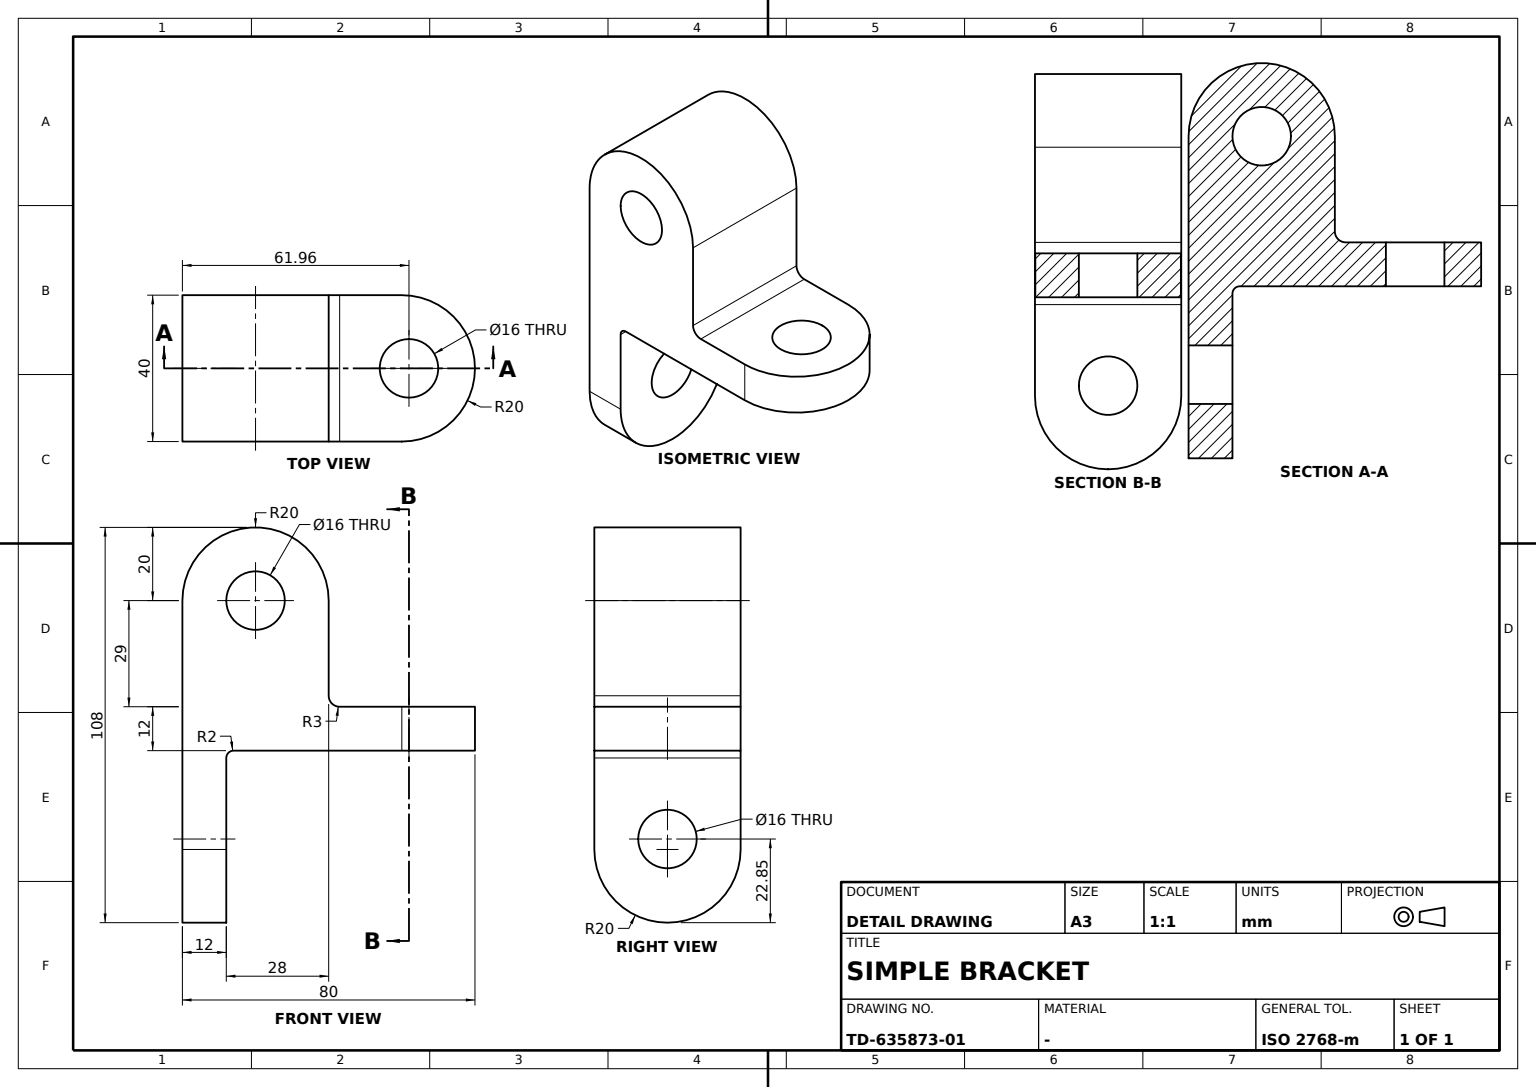
ISO-10303-21;
HEADER;
FILE_DESCRIPTION((''),'2;1');
FILE_NAME('','',(''),(''),'','','');
FILE_SCHEMA(('AUTOMOTIVE_DESIGN'));
ENDSEC;
DATA;
#1=APPLICATION_CONTEXT('');
#2=PRODUCT_CONTEXT('',#1,'mechanical');
#3=PRODUCT('','','',(#2));
#4=PRODUCT_DEFINITION_FORMATION('','',#3);
#5=PRODUCT_DEFINITION_CONTEXT('',#1,'design');
#6=PRODUCT_DEFINITION('','',#4,#5);
#7=PRODUCT_DEFINITION_SHAPE('','',#6);
#8=(LENGTH_UNIT()NAMED_UNIT(*)SI_UNIT(.MILLI.,.METRE.));
#9=(NAMED_UNIT(*)PLANE_ANGLE_UNIT()SI_UNIT($,.RADIAN.));
#10=(NAMED_UNIT(*)SI_UNIT($,.STERADIAN.)SOLID_ANGLE_UNIT());
#11=UNCERTAINTY_MEASURE_WITH_UNIT(LENGTH_MEASURE(1.E-05),#8,'distance_accuracy_value','');
#12=(GEOMETRIC_REPRESENTATION_CONTEXT(3)GLOBAL_UNCERTAINTY_ASSIGNED_CONTEXT((#11))GLOBAL_UNIT_ASSIGNED_CONTEXT((#8,#9,#10))REPRESENTATION_CONTEXT('',''));
#13=CARTESIAN_POINT('',(20.,20.,0.));
#14=VERTEX_POINT('',#13);
#15=CARTESIAN_POINT('',(20.,-20.,0.));
#16=VERTEX_POINT('',#15);
#17=CARTESIAN_POINT('',(20.,0.,0.));
#18=DIRECTION('',(1.,0.,0.));
#19=DIRECTION('',(0.,1.,0.));
#20=AXIS2_PLACEMENT_3D('',#17,#18,#19);
#21=CIRCLE('',#20,20.);
#22=EDGE_CURVE('',#14,#16,#21,.T.);
#23=ORIENTED_EDGE('',*,*,#22,.F.);
#24=CARTESIAN_POINT('',(-20.,20.,0.));
#25=VERTEX_POINT('',#24);
#26=CARTESIAN_POINT('',(0.,20.,0.));
#27=VECTOR('',#18,1000.);
#28=LINE('',#26,#27);
#29=EDGE_CURVE('',#25,#14,#28,.T.);
#30=ORIENTED_EDGE('',*,*,#29,.F.);
#31=CARTESIAN_POINT('',(-20.,-20.,0.));
#32=VERTEX_POINT('',#31);
#33=CARTESIAN_POINT('',(-20.,0.,0.));
#34=AXIS2_PLACEMENT_3D('',#33,#18,#19);
#35=CIRCLE('',#34,20.);
#36=EDGE_CURVE('',#25,#32,#35,.T.);
#37=ORIENTED_EDGE('',*,*,#36,.T.);
#38=CARTESIAN_POINT('',(0.,-20.,0.));
#39=LINE('',#38,#27);
#40=EDGE_CURVE('',#32,#16,#39,.T.);
#41=ORIENTED_EDGE('',*,*,#40,.T.);
#42=EDGE_LOOP('',(#23,#30,#37,#41));
#43=FACE_OUTER_BOUND('',#42,.T.);
#44=CARTESIAN_POINT('',(0.,0.,0.));
#45=DIRECTION('',(-1.,0.,0.));
#46=AXIS2_PLACEMENT_3D('',#44,#45,#19);
#47=CYLINDRICAL_SURFACE('',#46,20.);
#48=ADVANCED_FACE('',(#43),#47,.T.);
#49=CARTESIAN_POINT('',(-8.,-8.,-65.145943));
#50=VERTEX_POINT('',#49);
#51=CARTESIAN_POINT('',(-8.,-20.,-65.145943));
#52=VERTEX_POINT('',#51);
#53=CARTESIAN_POINT('',(-8.,-14.66,-65.145943));
#54=DIRECTION('',(0.,-1.,0.));
#55=VECTOR('',#54,1000.);
#56=LINE('',#53,#55);
#57=EDGE_CURVE('',#50,#52,#56,.T.);
#58=ORIENTED_EDGE('',*,*,#57,.T.);
#59=CARTESIAN_POINT('',(8.,-20.,-65.145943));
#60=VERTEX_POINT('',#59);
#61=CARTESIAN_POINT('',(0.,-20.,-65.145943));
#62=DIRECTION('',(0.,0.,-1.));
#63=AXIS2_PLACEMENT_3D('',#61,#54,#62);
#64=CIRCLE('',#63,8.);
#65=EDGE_CURVE('',#52,#60,#64,.T.);
#66=ORIENTED_EDGE('',*,*,#65,.T.);
#67=CARTESIAN_POINT('',(8.,-8.,-65.145943));
#68=VERTEX_POINT('',#67);
#69=CARTESIAN_POINT('',(8.,-14.66,-65.145943));
#70=LINE('',#69,#55);
#71=EDGE_CURVE('',#68,#60,#70,.T.);
#72=ORIENTED_EDGE('',*,*,#71,.F.);
#73=CARTESIAN_POINT('',(0.,-8.,-65.145943));
#74=AXIS2_PLACEMENT_3D('',#73,#19,#45);
#75=CIRCLE('',#74,8.);
#76=EDGE_CURVE('',#68,#50,#75,.T.);
#77=ORIENTED_EDGE('',*,*,#76,.T.);
#78=EDGE_LOOP('',(#58,#66,#72,#77));
#79=FACE_OUTER_BOUND('',#78,.T.);
#80=CARTESIAN_POINT('',(0.,-14.66,-65.145943));
#81=AXIS2_PLACEMENT_3D('',#80,#54,#45);
#82=CYLINDRICAL_SURFACE('',#81,8.);
#83=ADVANCED_FACE('',(#79),#82,.F.);
#84=CARTESIAN_POINT('',(-20.,20.,-26.));
#85=VERTEX_POINT('',#84);
#86=CARTESIAN_POINT('',(20.,20.,-26.));
#87=VERTEX_POINT('',#86);
#88=CARTESIAN_POINT('',(0.,20.,-26.));
#89=LINE('',#88,#27);
#90=EDGE_CURVE('',#85,#87,#89,.T.);
#91=ORIENTED_EDGE('',*,*,#90,.F.);
#92=CARTESIAN_POINT('',(-20.,20.,-13.));
#93=DIRECTION('',(0.,0.,1.));
#94=VECTOR('',#93,1000.);
#95=LINE('',#92,#94);
#96=EDGE_CURVE('',#85,#25,#95,.T.);
#97=ORIENTED_EDGE('',*,*,#96,.T.);
#98=ORIENTED_EDGE('',*,*,#29,.T.);
#99=CARTESIAN_POINT('',(20.,20.,-13.));
#100=LINE('',#99,#94);
#101=EDGE_CURVE('',#87,#14,#100,.T.);
#102=ORIENTED_EDGE('',*,*,#101,.F.);
#103=EDGE_LOOP('',(#91,#97,#98,#102));
#104=FACE_OUTER_BOUND('',#103,.T.);
#105=AXIS2_PLACEMENT_3D('',#26,#54,#62);
#106=PLANE('',#105);
#107=ADVANCED_FACE('',(#104),#106,.F.);
#108=ORIENTED_EDGE('',*,*,#65,.F.);
#109=EDGE_CURVE('',#60,#52,#64,.T.);
#110=ORIENTED_EDGE('',*,*,#109,.F.);
#111=EDGE_LOOP('',(#108,#110));
#112=FACE_BOUND('',#111,.T.);
#113=CARTESIAN_POINT('',(20.,-20.,-29.));
#114=VERTEX_POINT('',#113);
#115=CARTESIAN_POINT('',(20.,-20.,-68.));
#116=VERTEX_POINT('',#115);
#117=CARTESIAN_POINT('',(20.,-20.,-48.5));
#118=VECTOR('',#62,1000.);
#119=LINE('',#117,#118);
#120=EDGE_CURVE('',#114,#116,#119,.T.);
#121=ORIENTED_EDGE('',*,*,#120,.F.);
#122=CARTESIAN_POINT('',(-20.,-20.,-29.));
#123=VERTEX_POINT('',#122);
#124=CARTESIAN_POINT('',(0.,-20.,-29.));
#125=LINE('',#124,#27);
#126=EDGE_CURVE('',#123,#114,#125,.T.);
#127=ORIENTED_EDGE('',*,*,#126,.F.);
#128=CARTESIAN_POINT('',(-20.,-20.,-68.));
#129=VERTEX_POINT('',#128);
#130=CARTESIAN_POINT('',(-20.,-20.,-48.5));
#131=LINE('',#130,#118);
#132=EDGE_CURVE('',#123,#129,#131,.T.);
#133=ORIENTED_EDGE('',*,*,#132,.T.);
#134=CARTESIAN_POINT('',(0.,-20.,-88.));
#135=VERTEX_POINT('',#134);
#136=CARTESIAN_POINT('',(0.,-20.,-68.));
#137=AXIS2_PLACEMENT_3D('',#136,#19,#62);
#138=CIRCLE('',#137,20.);
#139=EDGE_CURVE('',#135,#129,#138,.T.);
#140=ORIENTED_EDGE('',*,*,#139,.F.);
#141=EDGE_CURVE('',#116,#135,#138,.T.);
#142=ORIENTED_EDGE('',*,*,#141,.F.);
#143=EDGE_LOOP('',(#121,#127,#133,#140,#142));
#144=FACE_OUTER_BOUND('',#143,.T.);
#145=AXIS2_PLACEMENT_3D('',#38,#54,#62);
#146=PLANE('',#145);
#147=ADVANCED_FACE('',(#112,#144),#146,.T.);
#148=CARTESIAN_POINT('',(20.,40.,-41.));
#149=VERTEX_POINT('',#148);
#150=CARTESIAN_POINT('',(0.,60.,-41.));
#151=VERTEX_POINT('',#150);
#152=CARTESIAN_POINT('',(0.,40.,-41.));
#153=AXIS2_PLACEMENT_3D('',#152,#93,#19);
#154=CIRCLE('',#153,20.);
#155=EDGE_CURVE('',#149,#151,#154,.T.);
#156=ORIENTED_EDGE('',*,*,#155,.T.);
#157=CARTESIAN_POINT('',(0.,60.,-29.));
#158=VERTEX_POINT('',#157);
#159=CARTESIAN_POINT('',(0.,60.,-34.));
#160=LINE('',#159,#94);
#161=EDGE_CURVE('',#151,#158,#160,.T.);
#162=ORIENTED_EDGE('',*,*,#161,.T.);
#163=CARTESIAN_POINT('',(20.,40.,-29.));
#164=VERTEX_POINT('',#163);
#165=CARTESIAN_POINT('',(0.,40.,-29.));
#166=AXIS2_PLACEMENT_3D('',#165,#62,#19);
#167=CIRCLE('',#166,20.);
#168=EDGE_CURVE('',#158,#164,#167,.T.);
#169=ORIENTED_EDGE('',*,*,#168,.T.);
#170=CARTESIAN_POINT('',(20.,40.,-35.));
#171=LINE('',#170,#94);
#172=EDGE_CURVE('',#149,#164,#171,.T.);
#173=ORIENTED_EDGE('',*,*,#172,.F.);
#174=EDGE_LOOP('',(#156,#162,#169,#173));
#175=FACE_OUTER_BOUND('',#174,.T.);
#176=CARTESIAN_POINT('',(0.,40.,-34.));
#177=AXIS2_PLACEMENT_3D('',#176,#93,#19);
#178=CYLINDRICAL_SURFACE('',#177,20.);
#179=ADVANCED_FACE('',(#175),#178,.T.);
#180=CARTESIAN_POINT('',(-8.,41.955551,-41.));
#181=VERTEX_POINT('',#180);
#182=CARTESIAN_POINT('',(8.,41.955551,-41.));
#183=VERTEX_POINT('',#182);
#184=CARTESIAN_POINT('',(0.,41.955551,-41.));
#185=AXIS2_PLACEMENT_3D('',#184,#62,#19);
#186=CIRCLE('',#185,8.);
#187=EDGE_CURVE('',#181,#183,#186,.T.);
#188=ORIENTED_EDGE('',*,*,#187,.F.);
#189=EDGE_CURVE('',#183,#181,#186,.T.);
#190=ORIENTED_EDGE('',*,*,#189,.F.);
#191=EDGE_LOOP('',(#188,#190));
#192=FACE_BOUND('',#191,.T.);
#193=CARTESIAN_POINT('',(-20.,32.,-41.));
#194=VERTEX_POINT('',#193);
#195=CARTESIAN_POINT('',(20.,32.,-41.));
#196=VERTEX_POINT('',#195);
#197=CARTESIAN_POINT('',(0.,32.,-41.));
#198=LINE('',#197,#27);
#199=EDGE_CURVE('',#194,#196,#198,.T.);
#200=ORIENTED_EDGE('',*,*,#199,.F.);
#201=CARTESIAN_POINT('',(-20.,40.,-41.));
#202=VERTEX_POINT('',#201);
#203=CARTESIAN_POINT('',(-20.,36.,-41.));
#204=VECTOR('',#19,1000.);
#205=LINE('',#203,#204);
#206=EDGE_CURVE('',#194,#202,#205,.T.);
#207=ORIENTED_EDGE('',*,*,#206,.T.);
#208=EDGE_CURVE('',#151,#202,#154,.T.);
#209=ORIENTED_EDGE('',*,*,#208,.F.);
#210=ORIENTED_EDGE('',*,*,#155,.F.);
#211=CARTESIAN_POINT('',(20.,36.,-41.));
#212=LINE('',#211,#204);
#213=EDGE_CURVE('',#196,#149,#212,.T.);
#214=ORIENTED_EDGE('',*,*,#213,.F.);
#215=EDGE_LOOP('',(#200,#207,#209,#210,#214));
#216=FACE_OUTER_BOUND('',#215,.T.);
#217=CARTESIAN_POINT('',(0.,-6.,-41.));
#218=AXIS2_PLACEMENT_3D('',#217,#62,#19);
#219=PLANE('',#218);
#220=ADVANCED_FACE('',(#192,#216),#219,.T.);
#221=ORIENTED_EDGE('',*,*,#90,.T.);
#222=CARTESIAN_POINT('',(20.,23.,-29.));
#223=VERTEX_POINT('',#222);
#224=CARTESIAN_POINT('',(20.,23.,-26.));
#225=AXIS2_PLACEMENT_3D('',#224,#45,#19);
#226=CIRCLE('',#225,3.);
#227=EDGE_CURVE('',#223,#87,#226,.T.);
#228=ORIENTED_EDGE('',*,*,#227,.F.);
#229=CARTESIAN_POINT('',(-20.,23.,-29.));
#230=VERTEX_POINT('',#229);
#231=CARTESIAN_POINT('',(0.,23.,-29.));
#232=LINE('',#231,#27);
#233=EDGE_CURVE('',#230,#223,#232,.T.);
#234=ORIENTED_EDGE('',*,*,#233,.F.);
#235=CARTESIAN_POINT('',(-20.,23.,-26.));
#236=AXIS2_PLACEMENT_3D('',#235,#45,#19);
#237=CIRCLE('',#236,3.);
#238=EDGE_CURVE('',#230,#85,#237,.T.);
#239=ORIENTED_EDGE('',*,*,#238,.T.);
#240=EDGE_LOOP('',(#221,#228,#234,#239));
#241=FACE_OUTER_BOUND('',#240,.T.);
#242=CARTESIAN_POINT('',(0.,23.,-26.));
#243=AXIS2_PLACEMENT_3D('',#242,#45,#19);
#244=CYLINDRICAL_SURFACE('',#243,3.);
#245=ADVANCED_FACE('',(#241),#244,.F.);
#246=CARTESIAN_POINT('',(0.,-8.,-88.));
#247=VERTEX_POINT('',#246);
#248=CARTESIAN_POINT('',(0.,10.,-88.));
#249=LINE('',#248,#204);
#250=EDGE_CURVE('',#135,#247,#249,.T.);
#251=ORIENTED_EDGE('',*,*,#250,.T.);
#252=CARTESIAN_POINT('',(20.,-8.,-68.));
#253=VERTEX_POINT('',#252);
#254=CARTESIAN_POINT('',(0.,-8.,-68.));
#255=AXIS2_PLACEMENT_3D('',#254,#54,#62);
#256=CIRCLE('',#255,20.);
#257=EDGE_CURVE('',#247,#253,#256,.T.);
#258=ORIENTED_EDGE('',*,*,#257,.T.);
#259=CARTESIAN_POINT('',(20.,-14.,-68.));
#260=LINE('',#259,#204);
#261=EDGE_CURVE('',#116,#253,#260,.T.);
#262=ORIENTED_EDGE('',*,*,#261,.F.);
#263=ORIENTED_EDGE('',*,*,#141,.T.);
#264=EDGE_LOOP('',(#251,#258,#262,#263));
#265=FACE_OUTER_BOUND('',#264,.T.);
#266=CARTESIAN_POINT('',(0.,10.,-68.));
#267=AXIS2_PLACEMENT_3D('',#266,#54,#62);
#268=CYLINDRICAL_SURFACE('',#267,20.);
#269=ADVANCED_FACE('',(#265),#268,.T.);
#270=ORIENTED_EDGE('',*,*,#57,.F.);
#271=EDGE_CURVE('',#50,#68,#75,.T.);
#272=ORIENTED_EDGE('',*,*,#271,.T.);
#273=ORIENTED_EDGE('',*,*,#71,.T.);
#274=ORIENTED_EDGE('',*,*,#109,.T.);
#275=EDGE_LOOP('',(#270,#272,#273,#274));
#276=FACE_OUTER_BOUND('',#275,.T.);
#277=ADVANCED_FACE('',(#276),#82,.F.);
#278=ORIENTED_EDGE('',*,*,#139,.T.);
#279=CARTESIAN_POINT('',(-20.,-8.,-68.));
#280=VERTEX_POINT('',#279);
#281=CARTESIAN_POINT('',(-20.,-14.,-68.));
#282=LINE('',#281,#204);
#283=EDGE_CURVE('',#129,#280,#282,.T.);
#284=ORIENTED_EDGE('',*,*,#283,.T.);
#285=EDGE_CURVE('',#280,#247,#256,.T.);
#286=ORIENTED_EDGE('',*,*,#285,.T.);
#287=ORIENTED_EDGE('',*,*,#250,.F.);
#288=EDGE_LOOP('',(#278,#284,#286,#287));
#289=FACE_OUTER_BOUND('',#288,.T.);
#290=AXIS2_PLACEMENT_3D('',#266,#54,#45);
#291=CYLINDRICAL_SURFACE('',#290,20.);
#292=ADVANCED_FACE('',(#289),#291,.T.);
#293=CARTESIAN_POINT('',(-8.,41.955551,-29.));
#294=VERTEX_POINT('',#293);
#295=CARTESIAN_POINT('',(8.,41.955551,-29.));
#296=VERTEX_POINT('',#295);
#297=CARTESIAN_POINT('',(0.,41.955551,-29.));
#298=AXIS2_PLACEMENT_3D('',#297,#93,#18);
#299=CIRCLE('',#298,8.);
#300=EDGE_CURVE('',#294,#296,#299,.T.);
#301=ORIENTED_EDGE('',*,*,#300,.T.);
#302=CARTESIAN_POINT('',(8.,41.955551,-59.16));
#303=LINE('',#302,#118);
#304=EDGE_CURVE('',#296,#183,#303,.T.);
#305=ORIENTED_EDGE('',*,*,#304,.T.);
#306=ORIENTED_EDGE('',*,*,#189,.T.);
#307=CARTESIAN_POINT('',(-8.,41.955551,-59.16));
#308=LINE('',#307,#118);
#309=EDGE_CURVE('',#294,#181,#308,.T.);
#310=ORIENTED_EDGE('',*,*,#309,.F.);
#311=EDGE_LOOP('',(#301,#305,#306,#310));
#312=FACE_OUTER_BOUND('',#311,.T.);
#313=CARTESIAN_POINT('',(0.,41.955551,-59.16));
#314=AXIS2_PLACEMENT_3D('',#313,#62,#18);
#315=CYLINDRICAL_SURFACE('',#314,8.);
#316=ADVANCED_FACE('',(#312),#315,.F.);
#317=CARTESIAN_POINT('',(-20.,40.,-29.));
#318=VERTEX_POINT('',#317);
#319=CARTESIAN_POINT('',(-20.,40.,-35.));
#320=LINE('',#319,#94);
#321=EDGE_CURVE('',#202,#318,#320,.T.);
#322=ORIENTED_EDGE('',*,*,#321,.T.);
#323=EDGE_CURVE('',#318,#158,#167,.T.);
#324=ORIENTED_EDGE('',*,*,#323,.T.);
#325=ORIENTED_EDGE('',*,*,#161,.F.);
#326=ORIENTED_EDGE('',*,*,#208,.T.);
#327=EDGE_LOOP('',(#322,#324,#325,#326));
#328=FACE_OUTER_BOUND('',#327,.T.);
#329=AXIS2_PLACEMENT_3D('',#176,#93,#45);
#330=CYLINDRICAL_SURFACE('',#329,20.);
#331=ADVANCED_FACE('',(#328),#330,.T.);
#332=ORIENTED_EDGE('',*,*,#76,.F.);
#333=ORIENTED_EDGE('',*,*,#271,.F.);
#334=EDGE_LOOP('',(#332,#333));
#335=FACE_BOUND('',#334,.T.);
#336=CARTESIAN_POINT('',(-20.,-8.,-43.));
#337=VERTEX_POINT('',#336);
#338=CARTESIAN_POINT('',(-20.,-8.,-55.5));
#339=LINE('',#338,#94);
#340=EDGE_CURVE('',#280,#337,#339,.T.);
#341=ORIENTED_EDGE('',*,*,#340,.T.);
#342=CARTESIAN_POINT('',(20.,-8.,-43.));
#343=VERTEX_POINT('',#342);
#344=CARTESIAN_POINT('',(0.,-8.,-43.));
#345=LINE('',#344,#27);
#346=EDGE_CURVE('',#337,#343,#345,.T.);
#347=ORIENTED_EDGE('',*,*,#346,.T.);
#348=CARTESIAN_POINT('',(20.,-8.,-55.5));
#349=LINE('',#348,#94);
#350=EDGE_CURVE('',#253,#343,#349,.T.);
#351=ORIENTED_EDGE('',*,*,#350,.F.);
#352=ORIENTED_EDGE('',*,*,#257,.F.);
#353=ORIENTED_EDGE('',*,*,#285,.F.);
#354=EDGE_LOOP('',(#341,#347,#351,#352,#353));
#355=FACE_OUTER_BOUND('',#354,.T.);
#356=AXIS2_PLACEMENT_3D('',#344,#54,#62);
#357=PLANE('',#356);
#358=ADVANCED_FACE('',(#335,#355),#357,.F.);
#359=ORIENTED_EDGE('',*,*,#40,.F.);
#360=CARTESIAN_POINT('',(-20.,-20.,-14.5));
#361=LINE('',#360,#118);
#362=EDGE_CURVE('',#32,#123,#361,.T.);
#363=ORIENTED_EDGE('',*,*,#362,.T.);
#364=ORIENTED_EDGE('',*,*,#126,.T.);
#365=CARTESIAN_POINT('',(20.,-20.,-14.5));
#366=LINE('',#365,#118);
#367=EDGE_CURVE('',#16,#114,#366,.T.);
#368=ORIENTED_EDGE('',*,*,#367,.F.);
#369=EDGE_LOOP('',(#359,#363,#364,#368));
#370=FACE_OUTER_BOUND('',#369,.T.);
#371=ADVANCED_FACE('',(#370),#146,.T.);
#372=CARTESIAN_POINT('',(-20.,-8.,0.));
#373=VERTEX_POINT('',#372);
#374=CARTESIAN_POINT('',(20.,-8.,0.));
#375=VERTEX_POINT('',#374);
#376=CARTESIAN_POINT('',(0.,-8.,0.));
#377=LINE('',#376,#27);
#378=EDGE_CURVE('',#373,#375,#377,.T.);
#379=ORIENTED_EDGE('',*,*,#378,.T.);
#380=CARTESIAN_POINT('',(20.,8.,0.));
#381=VERTEX_POINT('',#380);
#382=CIRCLE('',#20,8.);
#383=EDGE_CURVE('',#375,#381,#382,.T.);
#384=ORIENTED_EDGE('',*,*,#383,.T.);
#385=CARTESIAN_POINT('',(-20.,8.,0.));
#386=VERTEX_POINT('',#385);
#387=CARTESIAN_POINT('',(0.,8.,0.));
#388=LINE('',#387,#27);
#389=EDGE_CURVE('',#386,#381,#388,.T.);
#390=ORIENTED_EDGE('',*,*,#389,.F.);
#391=CIRCLE('',#34,8.);
#392=EDGE_CURVE('',#373,#386,#391,.T.);
#393=ORIENTED_EDGE('',*,*,#392,.F.);
#394=EDGE_LOOP('',(#379,#384,#390,#393));
#395=FACE_OUTER_BOUND('',#394,.T.);
#396=CYLINDRICAL_SURFACE('',#46,8.);
#397=ADVANCED_FACE('',(#395),#396,.F.);
#398=EDGE_CURVE('',#296,#294,#299,.T.);
#399=ORIENTED_EDGE('',*,*,#398,.T.);
#400=ORIENTED_EDGE('',*,*,#309,.T.);
#401=ORIENTED_EDGE('',*,*,#187,.T.);
#402=ORIENTED_EDGE('',*,*,#304,.F.);
#403=EDGE_LOOP('',(#399,#400,#401,#402));
#404=FACE_OUTER_BOUND('',#403,.T.);
#405=ADVANCED_FACE('',(#404),#315,.F.);
#406=ORIENTED_EDGE('',*,*,#392,.T.);
#407=EDGE_CURVE('',#386,#373,#391,.T.);
#408=ORIENTED_EDGE('',*,*,#407,.T.);
#409=EDGE_LOOP('',(#406,#408));
#410=FACE_BOUND('',#409,.T.);
#411=ORIENTED_EDGE('',*,*,#283,.F.);
#412=ORIENTED_EDGE('',*,*,#132,.F.);
#413=ORIENTED_EDGE('',*,*,#362,.F.);
#414=ORIENTED_EDGE('',*,*,#36,.F.);
#415=ORIENTED_EDGE('',*,*,#96,.F.);
#416=ORIENTED_EDGE('',*,*,#238,.F.);
#417=CARTESIAN_POINT('',(-20.,31.5,-29.));
#418=LINE('',#417,#55);
#419=EDGE_CURVE('',#318,#230,#418,.T.);
#420=ORIENTED_EDGE('',*,*,#419,.F.);
#421=ORIENTED_EDGE('',*,*,#321,.F.);
#422=ORIENTED_EDGE('',*,*,#206,.F.);
#423=CARTESIAN_POINT('',(-20.,-6.,-41.));
#424=VERTEX_POINT('',#423);
#425=CARTESIAN_POINT('',(-20.,13.,-41.));
#426=LINE('',#425,#204);
#427=EDGE_CURVE('',#424,#194,#426,.T.);
#428=ORIENTED_EDGE('',*,*,#427,.F.);
#429=CARTESIAN_POINT('',(-20.,-6.,-43.));
#430=AXIS2_PLACEMENT_3D('',#429,#45,#19);
#431=CIRCLE('',#430,2.);
#432=EDGE_CURVE('',#337,#424,#431,.T.);
#433=ORIENTED_EDGE('',*,*,#432,.F.);
#434=ORIENTED_EDGE('',*,*,#340,.F.);
#435=EDGE_LOOP('',(#411,#412,#413,#414,#415,#416,#420,#421,#422,#428,#433,#434));
#436=FACE_OUTER_BOUND('',#435,.T.);
#437=PLANE('',#34);
#438=ADVANCED_FACE('',(#410,#436),#437,.F.);
#439=ORIENTED_EDGE('',*,*,#383,.F.);
#440=EDGE_CURVE('',#381,#375,#382,.T.);
#441=ORIENTED_EDGE('',*,*,#440,.F.);
#442=EDGE_LOOP('',(#439,#441));
#443=FACE_BOUND('',#442,.T.);
#444=ORIENTED_EDGE('',*,*,#22,.T.);
#445=ORIENTED_EDGE('',*,*,#367,.T.);
#446=ORIENTED_EDGE('',*,*,#120,.T.);
#447=ORIENTED_EDGE('',*,*,#261,.T.);
#448=ORIENTED_EDGE('',*,*,#350,.T.);
#449=CARTESIAN_POINT('',(20.,-6.,-41.));
#450=VERTEX_POINT('',#449);
#451=CARTESIAN_POINT('',(20.,-6.,-43.));
#452=AXIS2_PLACEMENT_3D('',#451,#45,#19);
#453=CIRCLE('',#452,2.);
#454=EDGE_CURVE('',#343,#450,#453,.T.);
#455=ORIENTED_EDGE('',*,*,#454,.T.);
#456=CARTESIAN_POINT('',(20.,13.,-41.));
#457=LINE('',#456,#204);
#458=EDGE_CURVE('',#450,#196,#457,.T.);
#459=ORIENTED_EDGE('',*,*,#458,.T.);
#460=ORIENTED_EDGE('',*,*,#213,.T.);
#461=ORIENTED_EDGE('',*,*,#172,.T.);
#462=CARTESIAN_POINT('',(20.,31.5,-29.));
#463=LINE('',#462,#55);
#464=EDGE_CURVE('',#164,#223,#463,.T.);
#465=ORIENTED_EDGE('',*,*,#464,.T.);
#466=ORIENTED_EDGE('',*,*,#227,.T.);
#467=ORIENTED_EDGE('',*,*,#101,.T.);
#468=EDGE_LOOP('',(#444,#445,#446,#447,#448,#455,#459,#460,#461,#465,#466,#467));
#469=FACE_OUTER_BOUND('',#468,.T.);
#470=PLANE('',#20);
#471=ADVANCED_FACE('',(#443,#469),#470,.T.);
#472=ORIENTED_EDGE('',*,*,#427,.T.);
#473=ORIENTED_EDGE('',*,*,#199,.T.);
#474=ORIENTED_EDGE('',*,*,#458,.F.);
#475=LINE('',#217,#27);
#476=EDGE_CURVE('',#424,#450,#475,.T.);
#477=ORIENTED_EDGE('',*,*,#476,.F.);
#478=EDGE_LOOP('',(#472,#473,#474,#477));
#479=FACE_OUTER_BOUND('',#478,.T.);
#480=ADVANCED_FACE('',(#479),#219,.T.);
#481=ORIENTED_EDGE('',*,*,#440,.T.);
#482=ORIENTED_EDGE('',*,*,#378,.F.);
#483=ORIENTED_EDGE('',*,*,#407,.F.);
#484=ORIENTED_EDGE('',*,*,#389,.T.);
#485=EDGE_LOOP('',(#481,#482,#483,#484));
#486=FACE_OUTER_BOUND('',#485,.T.);
#487=ADVANCED_FACE('',(#486),#396,.F.);
#488=ORIENTED_EDGE('',*,*,#168,.F.);
#489=ORIENTED_EDGE('',*,*,#323,.F.);
#490=ORIENTED_EDGE('',*,*,#419,.T.);
#491=ORIENTED_EDGE('',*,*,#233,.T.);
#492=ORIENTED_EDGE('',*,*,#464,.F.);
#493=EDGE_LOOP('',(#488,#489,#490,#491,#492));
#494=FACE_OUTER_BOUND('',#493,.T.);
#495=ORIENTED_EDGE('',*,*,#300,.F.);
#496=ORIENTED_EDGE('',*,*,#398,.F.);
#497=EDGE_LOOP('',(#495,#496));
#498=FACE_BOUND('',#497,.T.);
#499=AXIS2_PLACEMENT_3D('',#231,#62,#19);
#500=PLANE('',#499);
#501=ADVANCED_FACE('',(#494,#498),#500,.F.);
#502=ORIENTED_EDGE('',*,*,#432,.T.);
#503=ORIENTED_EDGE('',*,*,#476,.T.);
#504=ORIENTED_EDGE('',*,*,#454,.F.);
#505=ORIENTED_EDGE('',*,*,#346,.F.);
#506=EDGE_LOOP('',(#502,#503,#504,#505));
#507=FACE_OUTER_BOUND('',#506,.T.);
#508=CARTESIAN_POINT('',(0.,-6.,-43.));
#509=AXIS2_PLACEMENT_3D('',#508,#45,#19);
#510=CYLINDRICAL_SURFACE('',#509,2.);
#511=ADVANCED_FACE('',(#507),#510,.F.);
#512=CLOSED_SHELL('',(#48,#83,#107,#147,#179,#220,#245,#269,#277,#292,#316,#331,#358,#371,#397,#405,#438,#471,#480,#487,#501,#511));
#513=MANIFOLD_SOLID_BREP('',#512);
#514=ADVANCED_BREP_SHAPE_REPRESENTATION('',(#513),#12);
#515=SHAPE_DEFINITION_REPRESENTATION(#7,#514);
ENDSEC;
END-ISO-10303-21;
